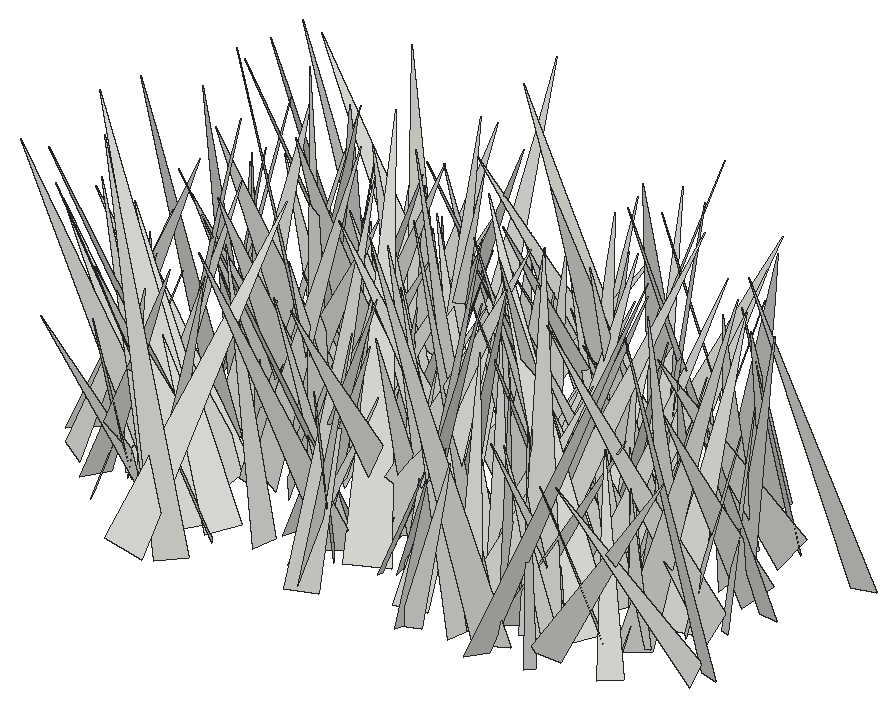
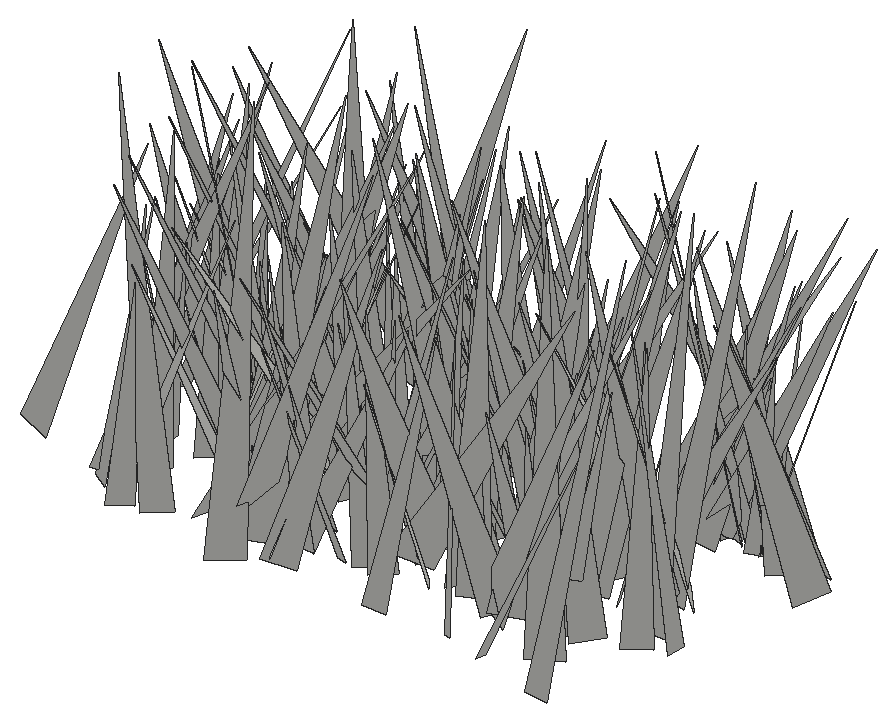
# SketchUp Ruby script. Lengths in inches.
U = 1.inch
M = Sketchup.active_model
def pt(a) = Geom::Point3d.new(a.map { |v| v * U })
def face(e, loops, mat)
  f = e.add_face(loops[0].map { |a| pt(a) })
  loops[1..].each { |l| e.add_face(l.map { |a| pt(a) }).erase! }
  f.material = f.back_material = mat if mat
  f
end
# faces: each face lists its corners as indices into pts; further lists are holes
def faces(e, pts, list, mat = nil) = list.each { |f| face(e, (f[0].is_a?(Array) ? f : [f]).map { |l| l.map { |i| pts[i] } }, mat) }
# xy, xz, yz: faces in a plane at the given z, y or x. An outline is a flat list of corners, or four numbers for a rectangle; further outlines are holes
def ring(l) = l.size == 4 ? [[l[0], l[1]], [l[2], l[1]], [l[2], l[3]], [l[0], l[3]]] : l.each_slice(2).to_a
def flat(e, list, mat, &to3) = list.each { |f| face(e, (f[0].is_a?(Array) ? f : [f]).map { |l| ring(l).map { |u, v| to3.(u, v) } }, mat) }
def xy(e, z, list, mat = nil) = flat(e, list, mat) { |x, y| [x, y, z] }
def xz(e, y, list, mat = nil) = flat(e, list, mat) { |x, z| [x, y, z] }
def yz(e, x, list, mat = nil) = flat(e, list, mat) { |y, z| [x, y, z] }
def lines(e, pts, list) = list.each { |a, b| e.add_line(pt(pts[a]), pt(pts[b])) }
# prism: a flat outline (further loops are holes) pulled along v
def prism(e, loops, v, mat = nil)
  f = face(e, loops, mat); d = Geom::Vector3d.new(v.map { |x| x * U })
  f.pushpull(f.normal.samedirection?(d) ? d.length : -d.length)
end
def box(e, o, s, mat = nil) = prism(e, [[o, [o[0] + s[0], o[1], o[2]], [o[0] + s[0], o[1] + s[1], o[2]], [o[0], o[1] + s[1], o[2]]]], [0, 0, s[2]], mat)
def at(x, y, z, deg = 0) = Geom::Transformation.translation(pt([x, y, z])) * Geom::Transformation.rotation(ORIGIN, Z_AXIS, deg.degrees)
def axes(o, x, y, z) = Geom::Transformation.new([*x, 0, *y, 0, *z, 0, *pt(o).to_a, 1])
def part(name) = M.definitions.add(name)
# library, detail: a bought-in or finely detailed component or shape, given as its bounding box
def library(name, o, s) = part(name).tap { |d| box(d.entities, o, s) }
def detail(e, o, s) = box(e.add_group.entities, o, s)
def put(e, d, t, mat = nil) = e.add_instance(d, t).tap { |i| i.material = mat if mat }
def group(e, t, mat = nil) = e.add_group.tap { |g| g.transformation = t; g.material = mat if mat }.entities
root = M.entities
c1 = part("fur_instance\#9")
p = [[0.8125,0,1.79],[0.67,-0.02,1.48],[0,-0.11,0],[0,0.11,0]]
faces(c1.entities,p,[[0,1,2,3]])
put(root,c1,axes([518.375,112.96,-21.86],[2.59266,-2.6088,0.97622],[-2.78019,-2.50569,0.68761],[-0.17141,1.18171,3.61316]))
put(root,c1,axes([508.91,111.2,-21.66],[-0.71343,7.62578,1.29035],[7.14993,0.15622,3.02994],[-2.94889,-1.46615,7.03427]))
put(root,c1,axes([521.49,113.67,-21.86],[-0.93338,-7.69941,2.7531],[-7.87622,0.10215,-2.38461],[-2.19672,2.90522,7.38009]))
put(root,c1,axes([503.76,115.7,-21.86],[-3.93384,-2.91751,0.42121],[-2.51987,3.69278,2.04402],[1.52955,-1.41982,4.45073]))
put(root,c1,axes([525.13,115.69,-21.66],[-2.98193,-4.15353,0.46379],[-3.81224,2.9367,1.78925],[1.71281,-0.69483,4.78981]))
put(root,c1,axes([508.95,113.45,-21.86],[-5.49378,-4.48735,0.1731],[-4.21573,5.05933,-2.64174],[-1.54724,2.14821,6.58325]))
put(root,c1,axes([523.67,113.98,-21.66],[3.57334,-4.4658,0.19156],[-4.12422,-3.19939,2.34597],[1.72363,1.60293,5.21618]))
put(root,c1,axes([507.09,110.74,-21.66],[-0.93463,7.10607,0.24964],[6.82555,0.96718,-1.97702],[1.99262,0.02006,6.88921]))
put(root,c1,axes([513.01,115.74,-21.86],[0.32689,-6.93131,1.01824],[-6.72809,-0.59471,-1.88835],[-1.95261,0.88881,6.67713]))
put(root,c1,axes([503.34,115.67,-21.86],[-2.16154,-4.08693,0.6496],[-3.73051,2.24163,1.68984],[1.79115,-0.26331,4.30345]))
put(root,c1,axes([502.71,114.67,-21.86],[5.28357,-2.5058,0.04843],[-2.504,-5.27298,0.35108],[0.10676,0.33794,5.83712]))
put(root,c1,axes([528.7,116.25,-21.66],[-4.92347,-1.39259,0.14711],[-1.23579,4.5738,1.93769],[0.65861,-1.82825,4.73553]))
put(root,c1,axes([512.87,115.49,-21.86],[-2.98653,-2.99705,1.42564],[-2.58075,3.30304,1.53746],[2.08674,-0.20437,3.94181]))
put(root,c1,axes([507.3,112.67,-21.66],[-6.47288,0.26814,0.01301],[0.25719,6.28405,-1.55397],[0.07694,1.55212,6.2893]))
put(root,c1,axes([513.8,112.69,-21.66],[4.21835,1.12148,1.8478],[0.48542,-4.44001,1.58659],[-2.10629,1.22277,4.06632]))
put(root,c1,axes([520.07,113.59,-21.86],[-6.43885,-0.2283,0.73687],[-0.34147,6.39798,-1.00159],[0.69173,1.03328,6.36457]))
put(root,c1,axes([505.89,115.125,-21.86],[-2.36054,6.29762,2.85628],[6.53149,1.03928,3.10644],[-2.27111,-3.55673,5.96508]))
put(root,c1,axes([507.35,115.84,-21.66],[-3.5976,-6.50533,0.64098],[-6.34012,3.29439,-2.15004],[-1.59153,1.58132,7.11613]))
put(root,c1,axes([505.85,116.43,-21.86],[0.77993,-5.26102,0.56712],[-5.12867,-0.89269,-1.22806],[-1.30258,0.36472,5.1748]))
put(root,c1,axes([503.54,113.48,-21.86],[4.04394,2.43918,0.42992],[2.39305,-4.06014,0.52577],[-0.63852,0.23141,4.69325]))
put(root,c1,axes([523.6,113.2,-21.86],[-4.31752,-0.25034,0.73123],[-0.52227,4.00392,-1.71296],[0.56974,1.77322,3.97108]))
put(root,c1,axes([515.63,116.43,-21.66],[7.87771,-0.03675,0.30438],[0.03502,-7.66773,-1.83222],[-0.30459,-1.83219,7.66177]))
put(root,c1,axes([523.375,114.78,-21.86],[-3.91396,0.19988,0.40503],[0.19284,3.93443,-0.07818],[0.40843,0.05784,3.91828]))
put(root,c1,axes([505.375,115.21,-21.86],[4.73571,-1.08461,0.9225],[-1.0987,-4.82145,-0.02851],[-0.90568,0.17765,4.85824]))
put(root,c1,axes([510.57,114.39,-21.86],[-5.56537,0.35389,1.01892],[0.25962,5.63719,-0.53984],[1.04691,0.48332,5.55042]))
put(root,c1,axes([518.17,112.93,-21.86],[6.62272,2.03005,2.53711],[1.31072,-6.93962,2.13125],[-2.97322,1.46257,6.59085]))
put(root,c1,axes([523.02,116.9,-21.86],[-4.32918,-1.79601,0.73607],[-1.48596,4.22424,1.56749],[1.24875,-1.19977,4.41706]))
put(root,c1,axes([506.1875,113.96,-21.86],[-5.02502,0.15502,0.9974],[-0.08895,4.97687,-1.22169],[1.00545,1.21508,4.87671]))
put(root,c1,axes([520.14,114.07,-21.86],[-0.91047,5.0165,1.03079],[5.11456,0.83694,0.44447],[-0.2628,-1.09133,5.07905]))
put(root,c1,axes([508.78,114.31,-21.86],[-3.94655,4.7323,0.06828],[4.56087,3.77904,1.70056],[-1.26405,-1.13963,5.92267]))
put(root,c1,axes([510.91,115.99,-21.86],[6.16535,-1.94029,0.16764],[-1.94054,-6.16752,-0.01601],[-0.16472,0.03505,6.46343]))
put(root,c1,axes([526.3125,114.38,-21.86],[-2.51117,3.39602,0.58609],[3.43959,2.51478,0.1658],[0.21361,-0.57041,4.22035]))
put(root,c1,axes([507.98,114.06,-21.86],[-4.22364,6.9226,0.63988],[6.72709,3.88063,2.42031],[-1.75445,-1.78585,7.73974]))
put(root,c1,axes([521.68,112.6,-21.66],[7.63616,1.08232,1.22596],[0.61242,-7.3209,2.64853],[-1.51635,2.49367,7.24345]))
put(root,c1,axes([505.67,115.75,-21.66],[-4.20776,3.77593,1.0344],[3.85861,3.7428,2.0336],[-0.66241,-2.18328,5.27517]))
put(root,c1,axes([513.84,118.75,-21.86],[6.11084,-2.63091,1.80363],[-1.49433,-5.80472,-3.40432],[-2.81811,-2.62692,5.71618]))
put(root,c1,axes([502.34,116.42,-21.86],[2.04033,-4.0488,0.48109],[-4.03745,-1.93127,0.8697],[0.56854,0.81522,4.44965]))
put(root,c1,axes([522.54,115.14,-21.86],[1.64686,-6.77743,3.62945],[-7.62252,-1.92308,-0.13234],[-1.0018,3.49096,6.97339]))
put(root,c1,axes([512.74,113.46,-21.66],[-3.04551,1.64304,1.0176],[0.80196,2.80235,-2.12461],[1.7584,1.56764,2.73144]))
put(root,c1,axes([511.29,116.38,-21.86],[4.36325,-2.68491,0.18726],[-2.69098,-4.34538,0.39756],[0.04948,0.43666,5.1077]))
put(root,c1,axes([513.96,112.27,-21.66],[-7.01528,2.7432,0.95764],[2.14491,6.5776,-3.12905],[1.96,2.6204,6.85188]))
put(root,c1,axes([504.19,115.46,-21.86],[3.4737,5.90005,1.74495],[6.11319,-3.08303,-1.74525],[0.69596,-2.36778,6.62052]))
put(root,c1,axes([521,115.1875,-21.86],[4.72114,-1.50275,0.05764],[-1.46013,-4.53503,1.361],[0.36002,1.31378,4.76394]))
put(root,c1,axes([505.17,115.03,-21.86],[5.7382,5.20942,1.87337],[5.41352,-5.84467,-0.3291],[-1.15821,-1.50876,7.74318]))
put(root,c1,axes([525.7,116.79,-21.86],[1.81522,-3.21568,0.8696],[-3.29805,-1.87418,-0.04607],[-0.46866,0.73395,3.69235]))
put(root,c1,axes([503.61,115.38,-21.86],[-2.88957,-1.62735,2.00469],[-2.2228,3.09866,-0.68855],[1.31385,1.66334,3.24403]))
put(root,c1,axes([520.13,117.28,-21.86],[4.34491,0.59069,1.09524],[0.90101,-4.23706,-1.28924],[-0.85828,-1.45776,4.19106]))
put(root,c1,axes([503.83,115.74,-21.86],[-2.18486,3.79279,1.02862],[3.92891,2.13324,0.47945],[0.08359,-1.13179,4.35074]))
put(root,c1,axes([514.9,118.11,-21.86],[2.86729,-4.50295,0.62999],[-4.43501,-2.93396,-0.78577],[-1.00209,0.10064,5.2802]))
put(root,c1,axes([529.16,116.4375,-21.66],[-3.64938,-5.29226,1.74557],[-5.55344,3.28039,-1.66476],[-0.463,2.36729,6.20923]))
put(root,c1,axes([501.1,115.39,-21.86],[2.45412,4.72767,0.6627],[4.74881,-2.3413,-0.8831],[0.48874,-0.99004,5.25297]))
put(root,c1,axes([516.14,117.66,-21.86],[1.75802,-6.33898,1.96931],[-6.51413,-2.03906,-0.74828],[-1.27556,1.67662,6.53555]))
put(root,c1,axes([512.32,117.18,-21.66],[-4.6508,-5.63712,0.37429],[-5.36466,4.25457,-2.58191],[-1.77136,1.91537,6.83673]))
put(root,c1,axes([527.18,119.28,-21.66],[-7.29024,-1.74958,0.87658],[-1.40156,7.02793,2.37084],[1.36568,-2.12702,7.11251]))
put(root,c1,axes([506.83,117.56,-21.86],[-6.1435,0.43905,0.01492],[0.43419,6.03663,1.1429],[-0.06685,-1.14104,6.05221]))
put(root,c1,axes([517.56,113.97,-21.86],[-5.11664,3.91829,0.85035],[3.38571,4.96082,-2.48663],[2.14782,1.51438,5.94556]))
put(root,c1,axes([519.71,115.55,-21.86],[-6.96753,-1.64469,0.65915],[-1.76863,6.61713,-2.18437],[0.10697,2.27915,6.81763]))
put(root,c1,axes([511.94,116.92,-21.66],[-1.05055,-3.99645,1.56356],[-4.12582,0.49771,-1.49997],[-1.18067,1.81677,3.85037]))
put(root,c1,axes([519.4375,117.07,-21.86],[4.14484,0.5886,1.74948],[0.68446,-4.48393,-0.11303],[-1.71425,-0.36717,4.1849]))
put(root,c1,axes([513.7,116.56,-21.66],[0.25719,7.17904,2.90731],[6.91163,1.10018,-3.3281],[3.49578,-2.70337,6.36621]))
put(root,c1,axes([500.28,117.05,-21.86],[6.2285,-2.9564,0.62521],[-3.02175,-6.08711,1.31964],[0.01382,1.46019,6.76705]))
put(root,c1,axes([522.68,118,-21.86],[-3.35511,-5.27651,0.83113],[-5.27558,3.11951,-1.49198],[-0.83701,1.48869,6.07225]))
put(root,c1,axes([515.52,119.16,-21.86],[7.4678,0.08394,0.57516],[0.2355,-7.21321,-2.00499],[-0.53141,-2.01703,7.1941]))
put(root,c1,axes([523.85,116.31,-21.86],[-7.18183,4.15456,0.03319],[4.14203,7.15453,0.70461],[-0.3242,-0.62648,8.26695]))
put(root,c1,axes([517.64,117.74,-21.86],[2.92691,3.10527,0.26779],[2.82947,-2.4932,-2.01476],[1.3071,-1.55642,3.76168]))
put(root,c1,axes([525.26,117.27,-21.86],[3.01506,-0.72225,2.0256],[-1.00024,-3.559,0.21985],[-1.90373,0.72607,3.09256]))
put(root,c1,axes([506.76,117.68,-21.86],[-4.43376,3.47486,0.22998],[3.34427,4.14468,1.85019],[-0.97128,-1.59146,5.32068]))
put(root,c1,axes([518.68,116.75,-21.86],[0.2906,4.64928,0.9365],[4.41539,0.07727,-1.75374],[1.73123,-0.9775,4.31562]))
put(root,c1,axes([508.71,118.08,-21.86],[3.8282,2.91024,0.83789],[3.01788,-3.55309,-1.44728],[0.25298,-1.65308,4.58585]))
put(root,c1,axes([511.52,116.27,-21.86],[4.39596,-0.31282,2.17467],[-1.10489,-4.51925,1.5834],[-1.89902,1.90528,4.11281]))
put(root,c1,axes([520.11,116.125,-21.86],[6.72656,-0.08852,1.07497],[-0.40385,-6.50233,1.99163],[-1.00015,2.03024,6.42556]))
put(root,c1,axes([525.68,116.5,-21.86],[6.60662,-2.19065,2.41659],[-2.83754,-6.55209,1.81792],[-1.6085,2.56075,6.71874]))
put(root,c1,axes([514.42,115.44,-21.86],[-3.14428,7.71271,0.49149],[7.72648,3.12546,0.38342],[-0.17032,-0.59964,8.32018]))
put(root,c1,axes([507.73,117.92,-21.66],[2.9133,6.77269,2.26525],[7.08174,-2.424,-1.8604],[0.9217,-2.7826,7.13411]))
put(root,c1,axes([507.59,121.18,-21.66],[5.40513,-4.44008,1.03103],[-3.91993,-5.34397,-2.46351],[-2.32626,-1.31164,6.54682]))
put(root,c1,axes([515.14,115.28,-21.86],[4.98815,3.01806,0.37753],[2.59556,-4.60182,2.49383],[-1.58564,1.9615,5.26983]))
put(root,c1,axes([504.25,120.2,-21.86],[-2.39726,-7.68863,1.50052],[-7.81274,2.46126,0.12966],[0.5725,1.39306,8.05265]))
put(root,c1,axes([520.07,120.61,-21.86],[0.49777,-7.47829,0.86543],[-7.52286,-0.52678,-0.22508],[-0.28353,0.84808,7.49146]))
put(root,c1,axes([518.65,117.6,-21.86],[-4.17339,1.81444,1.20525],[1.74242,4.34394,-0.50613],[1.30721,0.0026,4.52253]))
put(root,c1,axes([517.95,117.4,-21.86],[-7.81157,-0.92448,1.21309],[-1.13809,7.74743,-1.42443],[1.01538,1.5715,7.73604]))
put(root,c1,axes([509.9,119.79,-21.86],[-4.50462,1.14541,2.32905],[1.86637,4.67145,1.31236],[1.80364,-1.97324,4.45884]))
put(root,c1,axes([525.46,115.93,-21.86],[3.56764,3.88458,0.34534],[3.52617,-3.41301,1.96335],[-1.66594,1.09483,4.89523]))
put(root,c1,axes([516.57,119.89,-21.86],[-6.85321,0.30824,0.48855],[0.41589,6.6696,1.62593],[0.40091,-1.64973,6.66467]))
put(root,c1,axes([506.76,121.63,-21.86],[4.75153,-4.99406,0.9078],[-4.47168,-4.70683,-2.48828],[-2.40183,-1.11663,6.42854]))
put(root,c1,axes([518.12,117.43,-21.86],[-6.2227,2.39174,0.32304],[2.36421,6.22042,-0.51348],[0.48507,0.36431,6.64671]))
put(root,c1,axes([520.23,116.69,-21.86],[3.14457,7.68443,0.45621],[7.56933,-2.99688,-1.69436],[1.40136,-1.05601,8.12822]))
put(root,c1,axes([510.69,117.5,-21.86],[-8.04005,-0.21045,2.18635],[-0.63833,8.16213,-1.56173],[2.10165,1.67397,7.88972]))
put(root,c1,axes([525.04,119.8,-21.86],[0.27233,-6.25887,1.87066],[-6.53155,-0.29195,-0.02597],[-0.1084,1.8677,6.26474]))
put(root,c1,axes([526.68,122.3125,-21.86],[5.34512,-3.23236,0.64666],[-2.65449,-4.95104,-2.80671],[-1.95449,-2.11559,5.5804]))
put(root,c1,axes([514.9,119.87,-21.86],[-6.22259,1.31552,1.1088],[1.51746,6.15727,1.21077],[0.81078,-1.42761,6.24382]))
put(root,c1,axes([506.23,120.22,-21.66],[2.55754,-6.5759,0.86107],[-6.14173,-2.00015,2.96707],[2.50263,1.81158,6.40156]))
put(root,c1,axes([521.57,118.8,-21.86],[-6.43064,-2.17008,0.24743],[-2.17262,6.27662,-1.4168],[-0.22404,1.42068,6.6374]))
put(root,c1,axes([516.17,116.45,-21.86],[-7.73799,2.57835,1.8542],[1.9672,7.72518,-2.53263],[2.4932,1.90688,7.75308]))
put(root,c1,axes([514.2,120.41,-21.86],[1.97582,-3.11414,0.08334],[-3.10691,-1.9626,0.3224],[0.22782,0.24287,3.67393]))
put(root,c1,axes([526.21,118.73,-21.86],[2.95956,2.83712,0.75066],[2.89518,-2.997,-0.08741],[-0.48027,-0.58351,4.09885]))
put(root,c1,axes([515.8,120.89,-21.86],[-4.70083,-1.74871,0.0814],[-1.70109,4.61801,0.97093],[0.41342,-0.88228,4.92068]))
put(root,c1,axes([514.25,118.31,-21.86],[6.62959,-1.41825,2.66639],[-1.99694,-6.88369,1.30369],[-2.26567,1.91728,6.65307]))
put(root,c1,axes([521.875,120.47,-21.86],[-3.46593,0.7925,0.89611],[1.04093,3.35143,1.06213],[0.58952,-1.25841,3.39303]))
put(root,c1,axes([511.58,120.18,-21.86],[4.26328,-1.39926,0.74192],[-1.39292,-4.32659,-0.15583],[-0.75375,0.08115,4.48433]))
put(root,c1,axes([518.82,120.07,-21.86],[2.27684,-3.73592,1.683],[-3.94498,-2.51908,-0.25488],[-1.10756,1.29258,4.36763]))
put(root,c1,axes([522.41,117.69,-21.86],[2.81698,6.47491,0.35167],[6.46114,-2.77024,-0.75032],[0.54938,-0.62035,7.02117]))
put(root,c1,axes([506.96,118.67,-21.66],[2.66286,4.62658,1.9724],[4.32664,-3.24515,1.77077],[-2.56433,-0.67099,5.03592]))
put(root,c1,axes([525.82,118.54,-21.86],[-3.09006,5.24053,1.65653],[5.13422,3.43055,-1.27548],[1.9614,-0.72379,5.94851]))
put(root,c1,axes([508.78,120.48,-21.86],[-6.42891,-4.93695,1.78859],[-5.18873,6.40682,-0.96596],[0.80598,1.86616,8.04806]))
put(root,c1,axes([505.47,121.59,-21.86],[-3.15969,-2.10838,0.70871],[-1.88389,3.19122,1.09464],[1.18257,-0.54957,3.6374]))
put(root,c1,axes([516.52,120.96,-21.86],[4.31409,-4.88001,1.43702],[-5.06352,-4.30068,0.59646],[-0.49016,1.47666,6.48614]))
put(root,c1,axes([516.78,119.9,-21.86],[0.74077,3.76285,1.03817],[3.63302,-0.27816,-1.5841],[1.42759,-1.24465,3.49262]))
put(root,c1,axes([524.15,118.66,-21.86],[5.36611,5.59511,2.05394],[5.5109,-5.71038,1.15783],[-2.27022,-0.63666,7.66549]))
put(root,c1,axes([506.36,123.375,-21.66],[4.04445,-6.42376,0.8146],[-6.13253,-4.10829,-1.94934],[-2.07854,-0.37835,7.33638]))
put(root,c1,axes([522.5,119.92,-21.86],[4.29759,3.17988,0.45483],[3.21134,-4.23507,-0.73441],[0.07624,-0.86047,5.29543]))
put(root,c1,axes([522.21,121.51,-21.86],[0.21984,-5.04241,1.33274],[-4.72838,-0.75562,-2.0789],[-2.20101,1.11963,4.59917]))
put(root,c1,axes([519.4,119.35,-21.86],[0.34617,6.42334,1.62872],[6.51894,-0.03728,-1.2385],[1.18972,-1.66468,6.31231]))
put(root,c1,axes([512.58,120.97,-21.86],[-3.35147,5.54659,2.9979],[6.27053,3.28643,0.92965],[0.65767,-3.06906,6.41348]))
put(root,c1,axes([503.11,122.53,-21.86],[-1.7083,-7.51191,1.45388],[-7.48357,1.95063,1.28533],[1.59333,1.10775,7.59572]))
put(root,c1,axes([513.06,118.66,-21.86],[4.46685,2.95329,0.59597],[2.75098,-4.43263,1.34675],[-1.2285,0.81223,5.18275]))
put(root,c1,axes([523.4375,118.72,-21.86],[0.1109,6.16383,0.84068],[5.38265,-0.51661,3.07768],[-3.11876,-0.67243,5.34163]))
put(root,c1,axes([507.27,117.27,-21.66],[4.44404,5.53922,0.27989],[5.13876,-4.2472,2.46279],[-2.08674,1.3376,6.66087]))
put(root,c1,axes([508.41,120.31,-21.86],[6.24865,-3.61776,1.18124],[-3.80474,-5.99015,1.78079],[-0.08657,2.13519,6.99733]))
put(root,c1,axes([509.4,120.12,-21.86],[4.17015,5.48726,0.52169],[5.30168,-3.81404,-2.26221],[1.50809,-1.76505,6.51019]))
put(root,c1,axes([520.01,122.57,-21.66],[6.41369,-0.07562,0.05633],[-0.05586,-6.13403,-1.87481],[-0.07597,-1.87412,6.13403]))
put(root,c1,axes([523.32,122.7,-21.66],[5.23051,-1.10724,0.78196],[-0.81536,-5.06,-1.7109],[-1.08287,-1.53819,5.06527]))
put(root,c1,axes([528.1,121.11,-21.66],[-4.4516,-6.59475,1.62319],[-6.65602,3.85048,-2.61027],[-1.35017,2.76139,7.51625]))
put(root,c1,axes([504.47,120.35,-21.86],[-0.87926,6.56228,2.62812],[6.83144,1.46959,-1.38397],[1.81713,-2.34956,6.47466]))
put(root,c1,axes([509.06,123.28,-21.86],[-4.18199,-2.55213,0.91155],[-1.98836,4.02848,2.15666],[1.84139,-1.44616,4.39901]))
put(root,c1,axes([527.35,119.59,-21.86],[2.28996,3.33239,0.84649],[3.03653,-2.43723,1.38011],[-1.61271,0.14282,3.80053]))
put(root,c1,axes([507.82,121.3,-21.66],[4.10331,-3.61689,0.17449],[-3.47529,-3.85943,1.7253],[1.0172,1.40442,5.19061]))
put(root,c1,axes([507.82,124.72,-21.86],[5.60712,-6.07402,0.33398],[-5.83929,-5.5015,-2.02021],[-1.70529,-1.13347,8.01575]))
put(root,c1,axes([520.72,124.35,-21.66],[0.06912,-7.57158,0.2529],[-7.42195,-0.11839,-1.51598],[-1.51902,0.23392,7.41859]))
put(root,c1,axes([510.72,120.93,-21.86],[2.58495,3.56171,0.23056],[3.43761,-2.40789,-1.34382],[0.96012,-0.96809,4.1907]))
put(root,c1,axes([521.1,121.43,-21.86],[0.06663,3.86387,1.64805],[4.18879,0.06273,-0.31643],[0.31563,-1.6482,3.85147]))
put(root,c1,axes([512.73,122.46,-21.86],[5.22033,-0.21574,2.13038],[0.1303,-5.5713,-0.88347],[-2.13731,-0.86658,5.14955]))
put(root,c1,axes([520.83,123.42,-21.66],[5.55902,-2.83125,1.90418],[-2.404,-5.83322,-1.65498],[-2.42129,-0.70867,6.01496]))
put(root,c1,axes([503.61,119.69,-21.86],[4.49985,4.45709,1.03745],[4.28289,-4.6143,1.2473],[-1.61209,0.1822,6.20956]))
put(root,c1,axes([517.53,121.43,-21.86],[-4.36102,2.95909,2.58691],[3.11538,4.95832,-0.41976],[2.39639,-1.06094,5.25343]))
put(root,c1,axes([525.6875,125.51,-21.86],[5.96418,-2.86813,1.57613],[-1.66285,-5.47776,-3.67572],[-2.81874,-2.83722,5.50334]))
put(root,c1,axes([522.73,119.73,-21.86],[1.99959,6.47326,0.24716],[6.43471,-1.95494,-0.85747],[0.74746,-0.48749,6.72058]))
put(root,c1,axes([525.26,122.25,-21.86],[3.59976,0.06174,1.80471],[0.19659,-4.01441,-0.2548],[-1.79504,-0.31584,3.59126]))
put(root,c1,axes([516.51,120.86,-21.66],[1.26657,4.59176,1.22685],[4.36989,-1.62436,1.56816],[-1.86909,-0.68616,4.4977]))
put(root,c1,axes([501.72,123,-21.86],[5.83398,1.13984,1.03884],[1.35175,-5.73614,-1.2974],[-0.74243,-1.48703,5.80098]))
put(root,c1,axes([520.67,121.73,-21.86],[-5.00631,-5.98003,0.73957],[-5.22244,3.82659,-4.41068],[-3.00563,3.31169,6.43193]))
put(root,c1,axes([524.92,123.73,-21.66],[-1.49518,-5.85947,1.8909],[-5.5495,2.12534,2.19783],[2.66683,1.13753,5.63369]))
put(root,c1,axes([510.16,123.23,-21.86],[8.10386,-2.02713,0.06413],[-2.02706,-8.10412,-0.01624],[-0.06615,-0.00019,8.35354]))
put(root,c1,axes([504.42,124.625,-21.66],[8.18505,-1.50624,0.16494],[-1.43272,-7.98824,-1.85106],[-0.49323,-1.79175,8.11402]))
put(root,c1,axes([515.95,122.02,-21.86],[3.88682,0.49651,1.01606],[0.42112,-4.01087,0.34905],[-1.04955,0.22945,3.90283]))
put(root,c1,axes([502.89,123.75,-21.86],[3.52243,-4.25283,0.7835],[-4.27225,-3.57882,-0.21878],[-0.66956,0.46198,5.5178]))
put(root,c1,axes([520.6,120.53,-21.86],[-0.5351,4.97369,0.08314],[4.96853,0.53845,-0.2337],[0.24128,-0.05757,4.99693]))
put(root,c1,axes([524.4,124.2,-21.86],[5.38586,-3.00561,1.16634],[-2.8404,-5.49795,-1.05176],[-1.52519,-0.37466,6.07741]))
put(root,c1,axes([521.25,125.21,-21.66],[-3.70308,-3.24105,0.05421],[-3.08159,3.54543,1.46762],[1.00557,-1.07036,4.69716]))
put(root,c1,axes([515.83,122.02,-21.86],[-0.24087,4.17753,0.95098],[3.88217,0.61574,-1.72155],[1.81241,-0.76371,3.81393]))
put(root,c1,axes([506.35,123.85,-21.86],[6.51578,-0.90085,0.09034],[-0.89347,-6.50413,-0.41604],[-0.1463,-0.39981,6.56459]))
put(root,c1,axes([518.14,126.37,-21.66],[6.29678,-5.28708,1.00032],[-4.88133,-6.26054,-2.36253],[-2.26416,-1.20654,7.87535]))
put(root,c1,axes([520.51,123.97,-21.86],[-4.34148,-1.68145,0.56308],[-1.64517,4.37512,0.38015],[0.66161,-0.1544,4.64018]))
put(root,c1,axes([507.13,122.3,-21.86],[4.32331,2.64676,1.47041],[2.57631,-4.56233,0.63737],[-1.59061,-0.19566,5.02892]))
put(root,c1,axes([509.29,124.125,-21.66],[-4.9129,-5.75828,0.52895],[-5.68371,4.68095,-1.83254],[-1.06438,1.58274,7.34412]))
put(root,c1,axes([514.67,123.92,-21.86],[-6.25427,-0.78477,1.30734],[-0.71032,6.38344,0.43371],[1.34924,-0.27711,6.28838]))
put(root,c1,axes([520.83,125.89,-21.66],[-8.10416,-1.22815,0.06312],[-1.16757,7.81624,2.17553],[0.38615,-2.14192,7.90272]))
put(root,c1,axes([514.17,125.11,-21.86],[0.90872,-5.0896,0.45336],[-4.90772,-0.74115,1.51668],[1.42262,0.69427,4.94262]))
put(root,c1,axes([508.1,123.02,-21.86],[-2.49672,2.92464,0.96124],[2.97957,2.60694,-0.1927],[0.77439,-0.6012,3.84057]))
put(root,c1,axes([509.81,124.49,-21.86],[1.5026,-5.2869,1.47769],[-5.48951,-1.44343,0.41772],[0.01326,1.53554,5.48039]))
put(root,c1,axes([516.7,125.55,-21.66],[0.11807,-5.18176,0.38422],[-4.95689,-0.22756,-1.54584],[-1.55804,0.33133,4.94722]))
put(root,c1,axes([518.1875,123.48,-21.86],[-1.18817,5.57554,2.26119],[5.96275,1.39894,-0.31626],[0.80332,-2.13721,5.69196]))
put(root,c1,axes([529.51,124.78,-21.66],[-1.62801,-6.13851,1.48062],[-6.15059,1.19536,-1.80699],[-1.42958,1.84764,6.08822]))
put(root,c1,axes([505.57,124.72,-21.86],[-4.62696,1.13691,1.70574],[1.48296,4.76376,0.84751],[1.41525,-1.27471,4.68861]))
put(root,c1,axes([510.49,123.8,-21.86],[5.58768,-4.04107,3.86555],[-4.58295,-6.44048,-0.10822],[-3.20457,2.16447,6.89498]))
put(root,c1,axes([504.9375,126.42,-21.86],[1.80193,-7.44469,0.50754],[-7.36471,-1.69029,1.35351],[1.20089,0.80465,7.53912]))
put(root,c1,axes([517.17,126.86,-21.66],[-4.17954,-4.03403,0.06779],[-3.83281,4.00041,1.74723],[1.26,-1.21235,5.53978]))
put(root,c1,axes([519.65,120.14,-21.66],[5.70548,5.18554,0.14342],[4.71826,-5.27598,3.06024],[-2.15603,2.1765,7.07653]))
put(root,c1,axes([508.85,122.56,-21.86],[-4.46885,1.59045,1.08144],[1.18804,4.43404,-1.61169],[1.51249,1.21632,4.46123]))
put(root,c1,axes([522.47,122.64,-21.86],[4.1336,3.03674,0.5342],[2.87698,-4.11997,1.15876],[-1.10914,0.6308,4.99657]))
put(root,c1,axes([522.16,126.89,-21.66],[0.1957,-7.90399,1.09327],[-7.43409,0.21668,2.89722],[2.89871,1.0893,7.35646]))
put(root,c1,axes([512.96,124.04,-21.66],[-5.23637,6.32875,0.17784],[5.87309,4.76933,3.20385],[-2.36465,-2.16904,7.5636]))
put(root,c1,axes([513.02,123.83,-21.66],[2.725,5.40327,0.30402],[4.86473,-2.29653,-2.78814],[2.3711,-1.498,5.37096]))
put(root,c1,axes([513.32,125.11,-21.86],[3.01124,-3.84874,1.35887],[-4.04465,-3.04041,0.35153],[-0.54781,1.29229,4.87409]))
put(root,c1,axes([525.42,126.07,-21.86],[-3.17607,-4.40082,1.193],[-4.40846,3.33508,0.56622],[1.16445,0.62283,5.3976]))
put(root,c1,axes([516.64,126.91,-21.86],[2.95346,-5.37759,1.21149],[-5.08452,-3.18852,-1.75785],[-2.12927,0.1548,5.87804]))
put(root,c1,axes([518.35,127.81,-21.86],[7.64117,-3.1953,0.94942],[-2.87226,-7.51641,-2.18001],[-1.69158,-1.67105,7.9903]))
put(root,c1,axes([511.61,124.67,-21.86],[3.16954,2.48643,0.53995],[2.54162,-3.13416,-0.48689],[-0.1185,-0.71733,3.99891]))
put(root,c1,axes([516.36,125.74,-21.66],[-1.2496,-4.95098,2.04852],[-4.91628,1.89585,1.58307],[2.13046,1.47094,4.85465]))
put(root,c1,axes([519.625,124.1,-21.66],[0.86928,6.52033,1.58307],[6.24969,-0.2059,-2.58369],[2.44176,-1.79425,6.04937]))
put(root,c1,axes([524.72,125.31,-21.86],[-5.08452,-4.09315,0.88657],[-4.17476,4.84247,-1.58557],[-0.33349,1.78573,6.33184]))
put(root,c1,axes([517.23,123.4,-21.86],[1.99951,5.4557,0.6063],[5.41529,-2.06607,0.73224],[-0.89823,-0.31139,5.76424]))
put(root,c1,axes([518.89,126.15,-21.86],[-8.04315,1.60644,1.39343],[1.83623,7.99603,1.38066],[1.07265,-1.64234,8.08496]))
put(root,c1,axes([523.49,127.36,-21.66],[4.86782,-2.47433,0.4659],[-2.27673,-4.75873,-1.48527],[-1.07512,-1.1257,5.25471]))
put(root,c1,axes([508.75,127.21,-21.86],[-2.8265,-4.26887,1.57231],[-3.66111,3.23328,2.19698],[2.70032,-0.08465,4.62446]))
put(root,c1,axes([511.98,127.34,-21.86],[-0.22883,-5.12281,0.23524],[-5.12454,0.23734,0.18366],[0.19416,0.22665,5.12463]))
put(root,c1,axes([515.09,125.26,-21.86],[2.48404,3.35431,0.63876],[3.34518,-2.23213,-1.28736],[0.685,-1.26336,3.97047]))
put(root,c1,axes([508.59,124.92,-21.86],[-3.06653,-6.21678,2.70439],[-6.51984,1.89062,-3.04678],[-1.85842,3.62531,6.22648]))
put(root,c1,axes([508.37,124.71,-21.86],[-3.15581,4.82371,2.67558],[4.59437,4.00448,-1.80054],[3.05265,-1.04019,5.47589]))
put(root,c1,axes([520.94,123.16,-21.86],[0.42359,6.38348,0.10104],[6.1795,-0.43539,1.60081],[-1.60398,0.00839,6.194]))
put(root,c1,axes([503.3,128.96,-21.66],[-3.16063,-7.46069,0.64697],[-7.21635,3.22195,1.90087],[2.00118,-0.16476,7.87643]))
put(root,c1,axes([512.76,122.76,-21.86],[-6.29891,4.40553,1.36932],[3.82289,6.28157,-2.62437],[2.58248,1.44677,7.22479]))
put(root,c1,axes([506.88,127.6,-21.86],[-4.29176,-1.39668,0.34406],[-1.22552,4.11722,1.42648],[0.75311,-1.25938,4.28195]))
